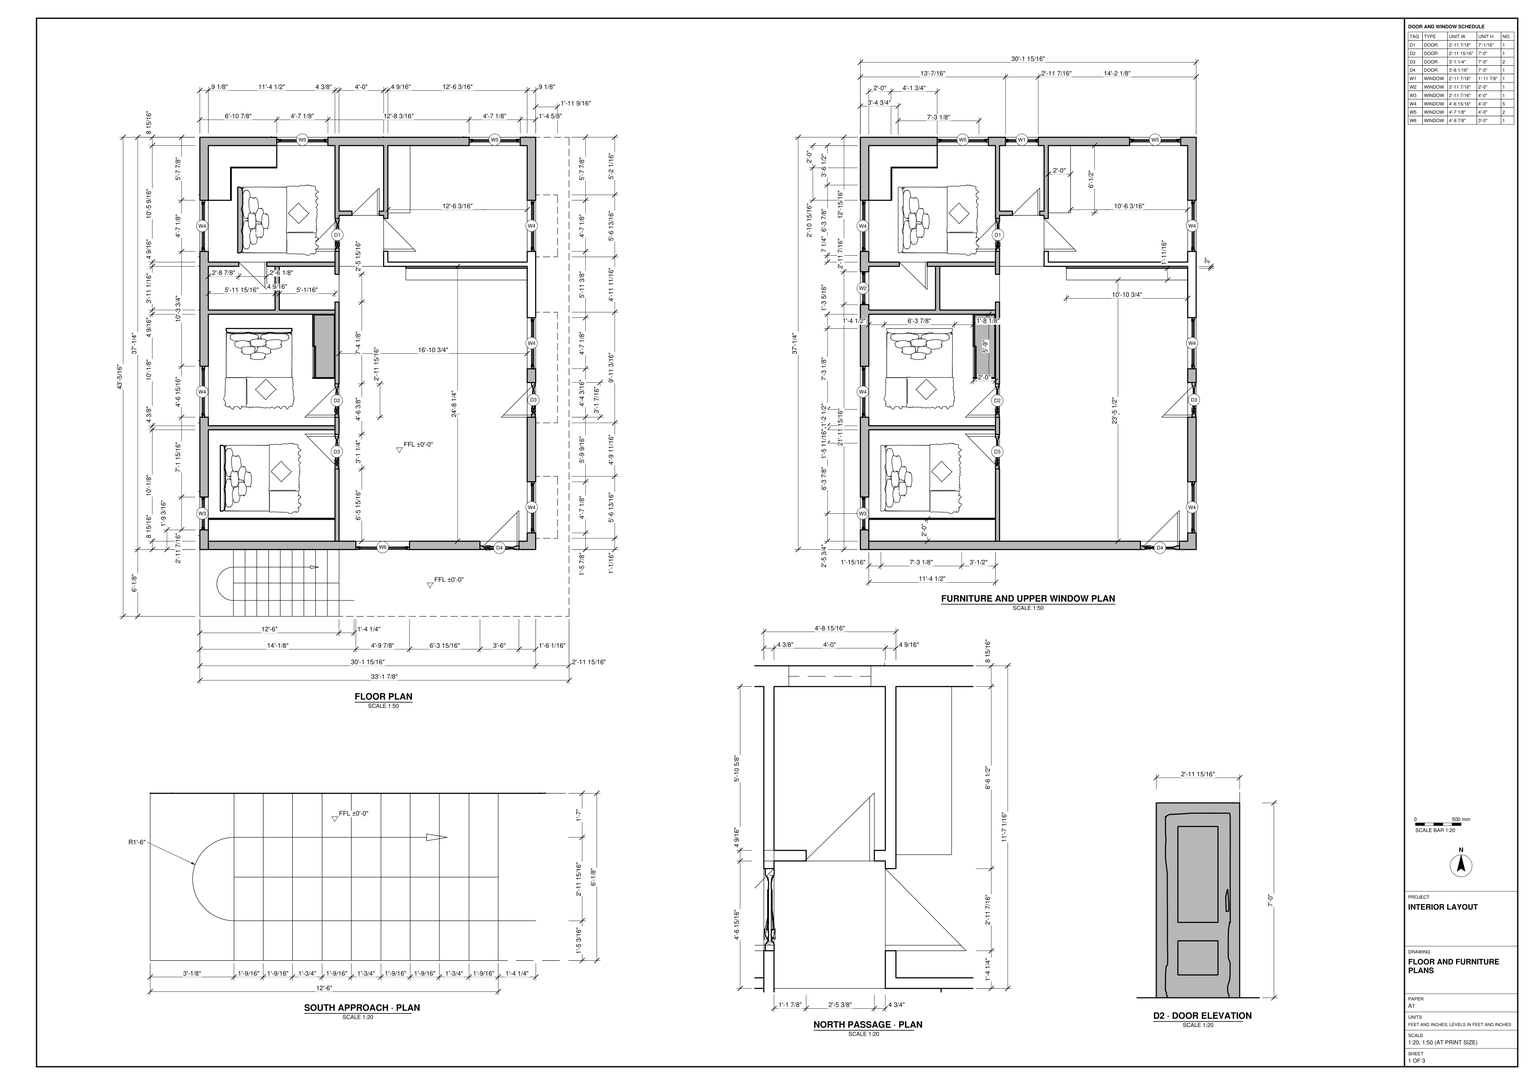
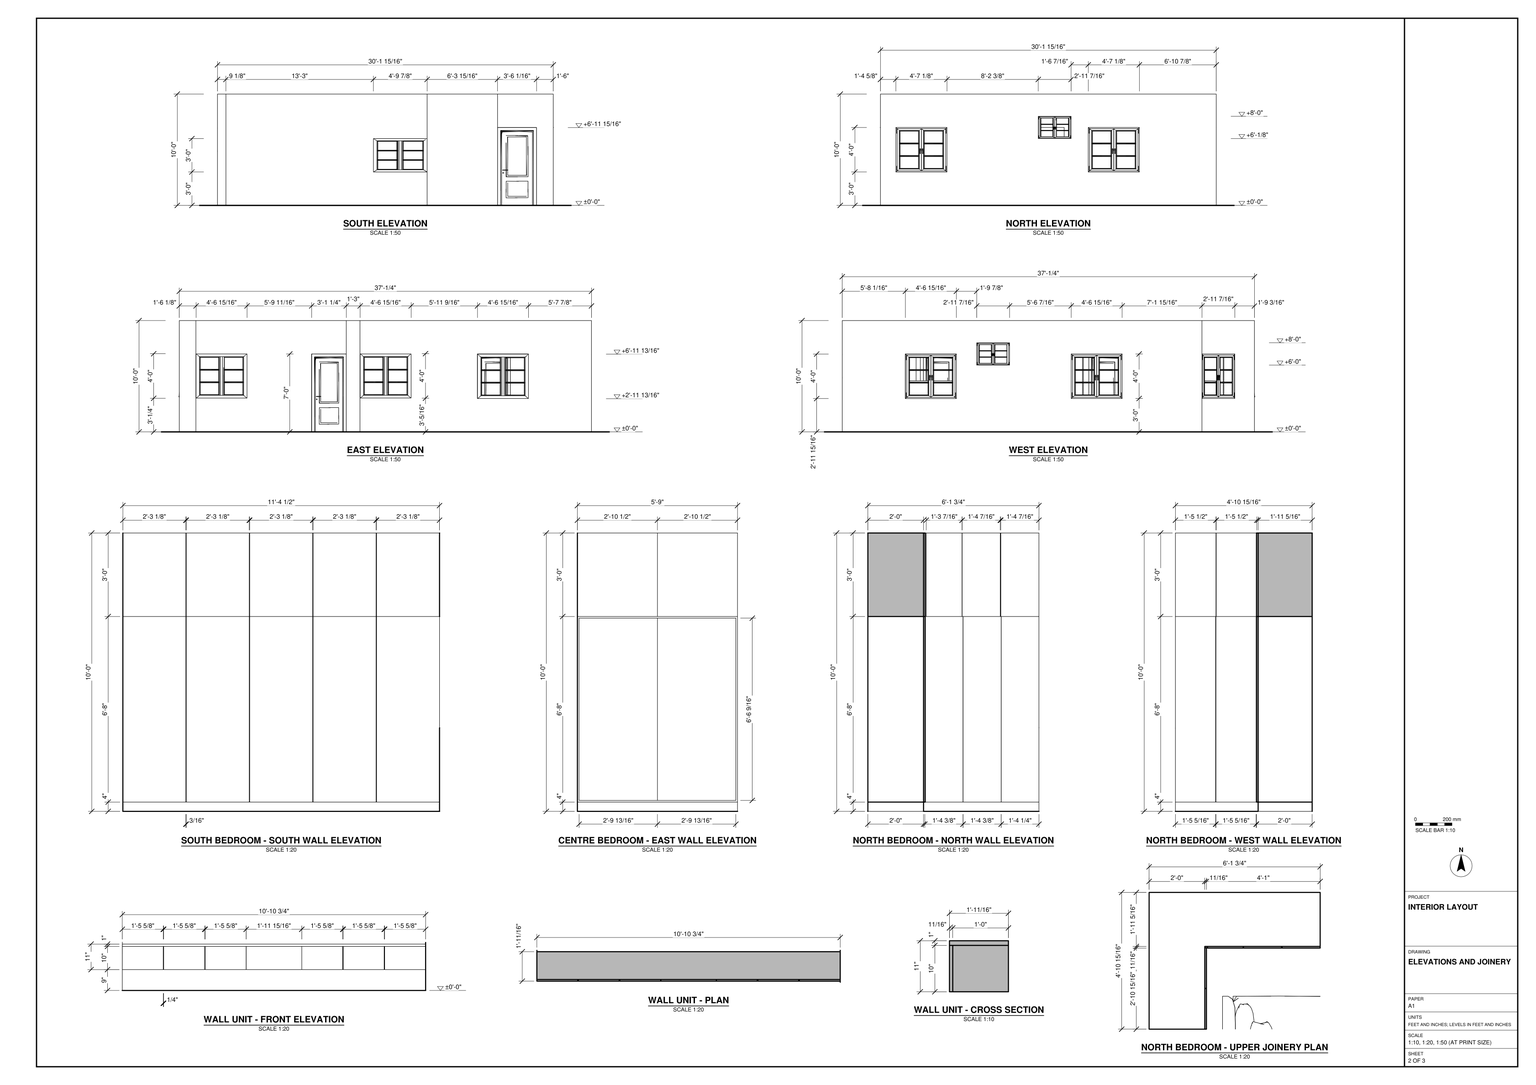
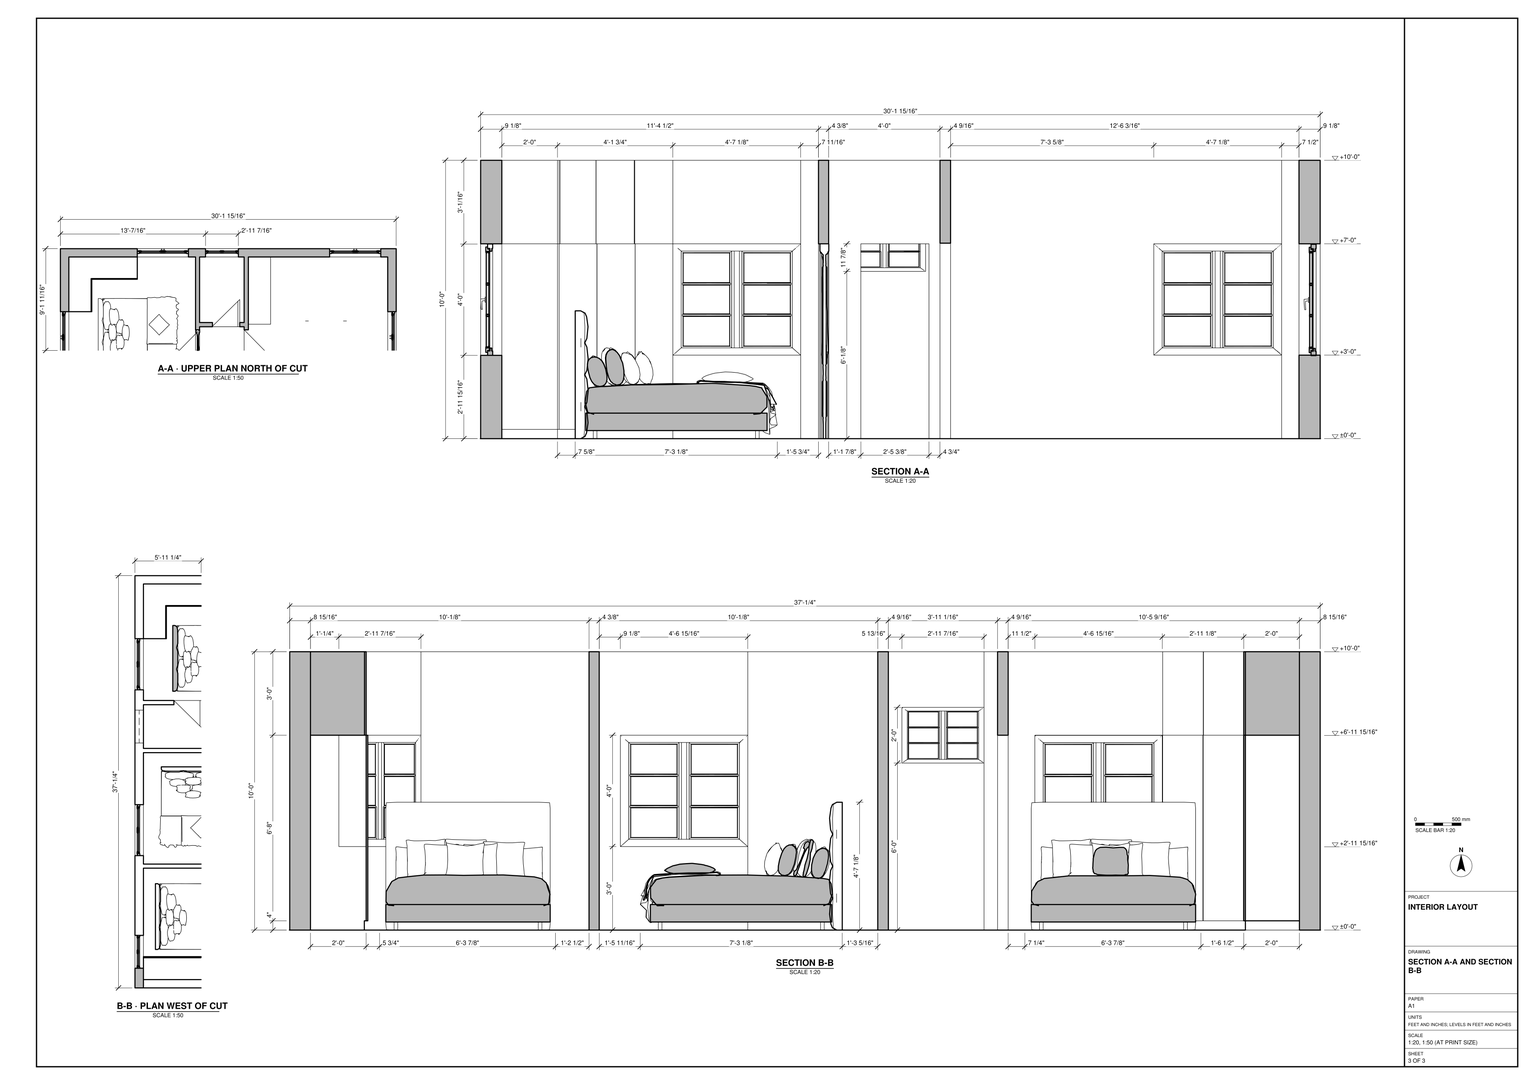
Build the single-storey interior in SketchUp from task_files/diagram_01.pdf. Work in feet and inches. The complete model extents are 120'-2 5/8" along X, 129'-1 1/8" along Y and 10'-1/16" along Z. These are not the room dimensions: use the dimensioned floor plan for the shell, which measures 30'-1 15/16" east to west by 37'-1/4" north to south. Set the finished floor level to ±0'-0".

Model the floor, perimeter walls and internal partitions using the individual wall thicknesses shown in plan. Arrange the three bedrooms along the west side, retaining the small space between the north and centre bedrooms, the narrow north passage and the large open room to the east. Include the divided south approach. Fit the doors and windows into wall openings; use the plans for door swings and the elevations and sections for sill heights, frames and window divisions. Note the smaller, higher windows on the north and west walls.

Place a bed in each bedroom with the footprint and orientation shown. Model the fitted storage along the south bedroom's south wall and the centre bedroom's east wall, and use the upper joinery plan for the corner storage in the north bedroom. Include the low wall unit in the large open room. Match the cabinet divisions to the joinery elevations. Decor and loose items may be any suitable library components.

Keep the shell elements and each furniture or joinery piece in separate groups or components, and use components for repeated parts. Save one SketchUp model as output_files/three_bedroom_interior_with_its_fitted_storage.skp.

# SketchUp Ruby script. Lengths in inches.
U = 1.inch
M = Sketchup.active_model
def pt(a) = Geom::Point3d.new(a.map { |v| v * U })
def face(e, loops, mat)
  f = e.add_face(loops[0].map { |a| pt(a) })
  loops[1..].each { |l| e.add_face(l.map { |a| pt(a) }).erase! }
  f.material = f.back_material = mat if mat
  f
end
# faces: each face lists its corners as indices into pts; further lists are holes
def faces(e, pts, list, mat = nil) = list.each { |f| face(e, (f[0].is_a?(Array) ? f : [f]).map { |l| l.map { |i| pts[i] } }, mat) }
# xy, xz, yz: faces in a plane at the given z, y or x. An outline is a flat list of corners, or four numbers for a rectangle; further outlines are holes
def ring(l) = l.size == 4 ? [[l[0], l[1]], [l[2], l[1]], [l[2], l[3]], [l[0], l[3]]] : l.each_slice(2).to_a
def flat(e, list, mat, &to3) = list.each { |f| face(e, (f[0].is_a?(Array) ? f : [f]).map { |l| ring(l).map { |u, v| to3.(u, v) } }, mat) }
def xy(e, z, list, mat = nil) = flat(e, list, mat) { |x, y| [x, y, z] }
def xz(e, y, list, mat = nil) = flat(e, list, mat) { |x, z| [x, y, z] }
def yz(e, x, list, mat = nil) = flat(e, list, mat) { |y, z| [x, y, z] }
def lines(e, pts, list) = list.each { |a, b| e.add_line(pt(pts[a]), pt(pts[b])) }
# prism: a flat outline (further loops are holes) pulled along v
def prism(e, loops, v, mat = nil)
  f = face(e, loops, mat); d = Geom::Vector3d.new(v.map { |x| x * U })
  f.pushpull(f.normal.samedirection?(d) ? d.length : -d.length)
end
def box(e, o, s, mat = nil) = prism(e, [[o, [o[0] + s[0], o[1], o[2]], [o[0] + s[0], o[1] + s[1], o[2]], [o[0], o[1] + s[1], o[2]]]], [0, 0, s[2]], mat)
def at(x, y, z, deg = 0) = Geom::Transformation.translation(pt([x, y, z])) * Geom::Transformation.rotation(ORIGIN, Z_AXIS, deg.degrees)
def axes(o, x, y, z) = Geom::Transformation.new([*x, 0, *y, 0, *z, 0, *pt(o).to_a, 1])
def part(name) = M.definitions.add(name)
# library, detail: a bought-in or finely detailed component or shape, given as its bounding box
def library(name, o, s) = part(name).tap { |d| box(d.entities, o, s) }
def detail(e, o, s) = box(e.add_group.entities, o, s)
def put(e, d, t, mat = nil) = e.add_instance(d, t).tap { |i| i.material = mat if mat }
def group(e, t, mat = nil) = e.add_group.tap { |g| g.transformation = t; g.material = mat if mat }.entities
root = M.entities
M.materials.add("[0007_MistyRose]").color = [255, 228, 225]
M.materials.add("[Basic Tile]").color = [203, 206, 207]
M.materials.add("[Color M00]").color = [255, 255, 255]
M.materials.add("[Concrete Tile]").color = [203, 190, 164]
M.materials.add("[Granite Tile]").color = [155, 148, 143]
M.materials.add("[Marble Carrara Gold Floor Tile]").color = [225, 223, 217]
M.materials.add("[Terrazzo Tile Accent]").color = [224, 221, 217]
c1 = part("29 cad.dwg")
xy(c1.entities,0,[[6.02,61.14,4.38,70.09,7.48,70.09],[174.3,112.79,174.3,115.72,183.25,114.26],[4.38,124.11,6.02,133.24,7.48,124.11],[6.02,133.24,4.38,142.18,7.48,142.18],[4.38,568.54,6.02,577.48,7.48,568.54],
  [823.51,569.27,826.98,569.82,830.45,569.27],[64.25,629.68,55.12,631.14,64.25,632.78],[407.92,629.68,407.92,632.78,417.05,631.14],[425.99,629.68,417.05,631.14,425.99,632.78],[444.0625,629.68,444.0625,632.78,453.01,631.14]])
# 826 loose lines left out
c2 = library("Bed 003",[-38.05,-87.1,0],[75.86,87.1,55.12])
c3 = library("Window 46-30",[-29.96,-2.6,0],[59.92,5.19,59.84])
c4 = library("Door 243 074",[-20.11,-2.41,0],[40.22,4.82,86.63])
c5 = part("Group\#6")
box(c5.entities,[0,0,0],[0.71,34.51,36])
c6 = part("Group\#13")
box(c6.entities,[0,0.16,0],[0.71,17.32,80])
c7 = part("Group\#14")
box(c7.entities,[0,1.07,0],[0.71,16.41,80])
c8 = part("Group\#18")
box(c8.entities,[0,0,0],[16.42,0.71,36])
c9 = part("Group\#17")
box(c9.entities,[-1.05,0,0],[17.47,0.71,36])
c10 = part("Group\#10")
box(c10.entities,[0,0,0],[17.64,0.71,10])
c11 = part("Group\#19")
box(c11.entities,[0.16,0,0],[27.14,0.71,80],"[Color M00]")
c12 = part("Group\#21")
box(c12.entities,[0.16,0,0],[27.14,0.71,36],"[Color M00]")
xy(root,0,[[398.98,439.99,417.05,439.99,417.05,582.53,407.92,582.53,407.92,448.93,398.98,448.93],[200.77,448.93,205.15,526.86],[55.12,496.57,64.25,496.57,64.25,569.03,200.77,569.03,200.77,573.41,64.25,573.41,64.25,637.47,55.12,637.47],[200.77,564.09,205.15,582.53],[200.77,618.49,205.15,706.64],
  [407.92,619.95,417.05,619.95,417.05,884.23,55.12,884.23,55.12,739.3125,64.25,739.3125,64.25,745.15,97.1,745.15,97.1,749.72,64.25,749.72,64.25,875.29,200.77,875.29,200.77,804.65,205.15,804.65,205.15,875.29,253.15,875.29,253.15,804.65,248.4,804.65,248.4,800.09,253.15,800.09,253.15,796.81,257.71,796.81,257.71,875.29,407.92,875.29,407.92,749.72,257.71,749.72,257.71,761.4,253.15,761.4,253.15,745.15,407.92,745.15],[176.77,624.49,200.77,693.5],[55.12,637.47,64.25,637.47,64.25,693.5,200.77,693.5,200.77,698.06,140.72,698.06,140.72,745.15,136.16,745.15,136.16,698.06,64.25,698.06,64.25,739.3125,55.12,739.3125],[200.77,736.58,205.15,761.4],[277.15,743.15,407.92,745.15],
  [127.21,745.15,200.77,749.72],[200.77,796.81,205.15,800.09],[200.77,800.09,205.15,804.65],[205.15,800.09,219.02,804.65]])
xy(root,0,[[[0,0,1442.625,1549.125],[398.98,439.99,398.98,448.93,64.25,448.93,64.25,472.93,200.77,472.93,200.77,526.86,205.15,526.86,205.15,564.09,200.77,564.09,200.77,569.03,64.25,569.03,64.25,496.57,55.12,496.57,55.12,884.23,417.05,884.23,417.05,619.95,407.92,619.95,407.92,582.53,417.05,582.53,417.05,439.99]]],"[0007_MistyRose]")
xy(root,0,[[64.25,749.72,200.77,749.72,200.77,875.29,137.98,875.29,137.98,852,88.25,852,88.25,816.34,64.25,816.34],[200.77,761.4,205.15,796.81]],"[Basic Tile]")
xy(root,0,[[64.25,448.93,200.77,472.93]],"[Color M00]")
xy(root,0,[[219.02,800.09,248.4,800.09,248.4,804.65,253.15,804.65,253.15,875.29,205.15,875.29,205.15,804.65,219.02,804.65]],"[Concrete Tile]")
xy(root,0,[[257.71,749.72,407.92,749.72,407.92,875.29,281.71,875.29,281.71,802.81,257.71,802.81,257.71,796.81,253.15,796.81,253.15,761.4,257.71,761.4],[257.71,802.81,281.71,875.29]],"[Granite Tile]")
xy(root,0,[[205.15,448.93,407.92,448.93,407.92,743.15,277.15,743.15,277.15,745.15,205.15,745.15],[205.15,745.15,253.15,800.09]],"[Marble Carrara Gold Floor Tile]")
xy(root,0,[[64.25,573.41,200.77,573.41,200.77,582.53,205.15,582.53,205.15,618.49,200.77,618.49,200.77,624.49,176.77,624.49,176.77,693.5,64.25,693.5],[64.25,698.06,136.16,698.06,136.16,745.15,127.21,745.15,127.21,749.72,97.1,749.72,97.1,745.15,64.25,745.15],[140.72,698.06,200.77,698.06,200.77,706.64,205.15,706.64,205.15,736.58,200.77,736.58,200.77,745.15,140.72,745.15]],"[Terrazzo Tile Accent]")
xy(root,4,[[64.25,816.34,64.25,875.29,137.98,875.29,137.98,852,88.25,852,88.25,816.34]])
xy(root,35.92,[[55.12,761.22,64.25,816.34]])
xy(root,36,[[55.12,582.53,64.25,637.47],[407.92,761.22,417.05,816.34],[137.98,875.29,193.1,884.23],[345.32,875.29,400.44,884.23]])
xy(root,36.44,[[407.92,457.875,417.05,512.99]])
xy(root,36.52,[[407.92,634.73,417.05,689.85]])
xy(root,72,[[55.12,703.91,64.25,739.3125]])
xy(root,72.11,[[211.54,875.29,246.94,884.23]])
xy(root,84,[[357,439.99,398.98,448.93],[407.92,457.875,417.05,512.99],[200.77,526.86,205.15,564.09],[55.12,582.53,64.25,637.47],[200.77,582.53,205.15,618.49],
  [407.92,582.53,417.05,619.95],[407.92,634.73,417.05,689.85],[200.77,706.64,205.15,736.58],[97.1,745.15,127.21,749.72],[127.21,745.15,136.16,749.72],
  [55.12,761.22,64.25,816.34],[407.92,761.22,417.05,816.34],[200.77,761.4,205.15,796.81],[219.02,800.09,248.4,804.65],[64.25,816.34,88.25,816.34,88.25,852,137.98,852,137.98,875.29,64.25,875.29],
  [137.98,875.29,193.1,884.23],[345.32,875.29,400.44,884.23]])
xy(root,84.27,[[253.15,761.4,257.71,796.81]])
xy(root,96,[[55.12,703.91,64.25,739.3125],[211.54,875.29,246.94,884.23]])
xy(root,120,[[[357,439.99,417.05,439.99,417.05,884.23,55.12,884.23,55.12,496.57,64.25,496.57,64.25,745.15,136.16,745.15,136.16,749.72,64.25,749.72,64.25,875.29,253.15,875.29,253.15,804.65,205.15,804.65,205.15,875.29,200.77,875.29,200.77,761.4,205.15,761.4,205.15,800.09,253.15,800.09,253.15,745.15,407.92,745.15,407.92,448.93,357,448.93],[257.71,749.72,407.92,875.29]],[200.77,448.93,205.15,582.53],[64.25,569.03,200.77,573.41],[200.77,582.53,205.15,761.4],[64.25,693.5,200.77,693.5,200.77,698.06,140.72,698.06,140.72,745.15,136.16,745.15,136.16,698.06,64.25,698.06],
  [277.28,743.15,407.92,745.15],[136.16,745.15,200.77,749.72]])
xz(root,439.99,[[398.98,0,417.05,0,417.05,120,357,120,357,84,398.98,84]])
xz(root,448.93,[[200.77,0,205.15,120],[398.98,0,398.98,84,357,84,357,120,407.92,120,407.92,0]])
xz(root,457.875,[[407.92,36.44,417.05,84]])
xz(root,496.57,[[55.12,0,64.25,120]])
xz(root,512.99,[[407.92,36.44,417.05,84]])
xz(root,526.86,[[200.77,0,205.15,84]])
xz(root,564.09,[[200.77,0,205.15,84]])
xz(root,569.03,[[64.25,0,200.77,120]])
xz(root,573.41,[[64.25,0,200.77,120]])
xz(root,582.53,[[200.77,0,205.15,84],[407.92,0,417.05,84],[55.12,36,64.25,84]])
xz(root,618.49,[[200.77,0,205.15,84]])
xz(root,619.95,[[407.92,0,417.05,84]])
xz(root,634.73,[[407.92,36.52,417.05,84]])
xz(root,637.47,[[55.12,36,64.25,84]])
xz(root,689.85,[[407.92,36.52,417.05,84]])
xz(root,693.5,[[64.25,0,200.77,120]])
xz(root,698.06,[[64.25,0,136.16,120],[140.72,0,200.77,120]])
xz(root,703.91,[[55.12,72,64.25,96]])
xz(root,706.64,[[200.77,0,205.15,84]])
xz(root,736.58,[[200.77,0,205.15,84]])
xz(root,737.15,[[407.92,87.4,407.92,88.4,277.25,88.55,277.25,87.55]])
xz(root,739.3125,[[55.12,72,64.25,96]])
xz(root,743.15,[[277.15,0,407.92,0,407.92,87.4,277.25,87.55],[407.92,88.4,407.92,120,277.28,120,277.25,88.55]])
xz(root,745.15,[[64.25,0,97.1,0,97.1,84,136.16,84,136.16,120,64.25,120],[127.21,0,136.16,84],[136.16,0,140.72,120],[140.72,0,200.77,120],[253.15,0,277.15,0,277.28,120,253.15,120],
  [277.15,0,277.28,120,407.92,120,407.92,0]])
xz(root,749.72,[[64.25,0,64.25,120,136.16,120,136.16,84,97.1,84,97.1,0],[127.21,0,127.21,84,136.16,84,136.16,120,200.77,120,200.77,0],[257.71,0,407.92,120]])
xz(root,761.22,[[55.12,35.92,64.25,84],[407.92,36,417.05,84]])
xz(root,761.4,[[200.77,0,205.15,84],[253.15,0,257.71,84.27]])
xz(root,796.81,[[200.77,0,205.15,84],[253.15,0,257.71,84.27]])
xz(root,800.09,[[205.15,0,219.02,0,219.02,84,248.4,84,248.4,0,253.15,0,253.15,120,205.15,120]])
xz(root,804.65,[[205.15,0,205.15,120,248.4,120,248.4,84,219.02,84,219.02,0],[248.4,0,253.15,120]])
xz(root,816.34,[[64.25,0,88.25,4],[64.25,4,88.25,84],[55.12,35.92,64.25,84],[407.92,36,417.05,84]])
xz(root,852,[[88.25,0,137.98,4],[88.25,4,104.82,84],[104.82,4,121.4,84],[121.4,4,137.98,84]])
xz(root,875.29,[[64.25,0,137.98,4],[137.98,0,193.1,36],[193.1,0,200.77,120],[[205.15,0,253.15,120],[211.54,72.11,246.94,96]],[257.71,0,400.44,0,400.44,36,345.32,36,345.32,84,400.44,84,400.44,120,257.71,120],
  [400.44,0,407.92,120],[64.25,4,137.98,84],[64.25,84,193.1,120]])
xz(root,884.23,[[[55.12,0,417.05,120],[137.98,36,193.1,84],[345.32,36,400.44,84],[211.54,72.11,246.94,96]]])
yz(root,55.12,[[[496.57,0,884.23,120],[761.22,35.92,816.34,84],[582.53,36,637.47,84],[703.91,72,739.3125,96]]])
yz(root,64.25,[[496.57,0,569.03,120],[573.41,0,637.47,0,637.47,36,582.53,36,582.53,84,637.47,84,637.47,120,573.41,120],[637.47,0,693.5,120],[698.06,0,739.3125,0,739.3125,72,703.91,72,703.91,96,739.3125,96,739.3125,120,698.06,120],[739.3125,0,745.15,120],
  [749.72,0,816.34,0,816.34,35.92,761.22,35.92,761.22,84,875.29,84,875.29,120,749.72,120],[816.34,0,875.29,4],[816.34,4,875.29,84]])
yz(root,88.25,[[816.34,0,852,4],[816.34,4,833.8125,84],[833.8125,4,852,84]])
yz(root,97.1,[[745.15,0,749.72,84]])
yz(root,127.21,[[745.15,0,749.72,84]])
yz(root,136.16,[[698.06,0,745.15,120],[745.15,84,749.72,120]])
yz(root,137.98,[[852,0,875.29,4],[852,4,875.29,84],[875.29,36,884.23,84]])
yz(root,140.72,[[698.06,0,745.15,120]])
yz(root,193.1,[[875.29,36,884.23,84]])
yz(root,200.77,[[448.93,0,448.93,120,569.03,120,569.03,0,564.09,0,564.09,84,526.86,84,526.86,0],[569.03,0,573.41,120],[573.41,0,582.53,120],[618.49,0,618.49,84,582.53,84,582.53,120,693.5,120,693.5,0],[693.5,0,698.06,120],
  [698.06,0,698.06,120,745.15,120,745.15,0,736.58,0,736.58,84,706.64,84,706.64,0],[745.15,0,749.72,120],[749.72,0,761.4,120],[796.81,0,796.81,84,761.4,84,761.4,120,800.09,120,800.09,0],[800.09,0,804.65,120],
  [804.65,0,875.29,120]])
yz(root,205.15,[[448.93,0,526.86,0,526.86,84,564.09,84,564.09,0,582.53,0,582.53,120,448.93,120],[618.49,0,706.64,0,706.64,84,736.58,84,736.58,0,761.4,0,761.4,120,582.53,120,582.53,84,618.49,84],[796.81,0,800.09,0,800.09,120,761.4,120,761.4,84,796.81,84],[804.65,0,875.29,120]])
yz(root,211.54,[[875.29,72.11,884.23,96]])
yz(root,219.02,[[800.09,0,804.65,84]])
yz(root,246.94,[[875.29,72.11,884.23,96]])
yz(root,248.4,[[800.09,0,804.65,84]])
yz(root,253.15,[[745.15,0,745.15,120,800.09,120,800.09,0,796.81,0,796.81,84.27,761.4,84.27,761.4,0],[804.65,0,875.29,120]])
yz(root,257.71,[[749.72,0,761.4,0,761.4,84.27,796.81,84.27,796.81,0,875.29,0,875.29,120,749.72,120]])
yz(root,277.25,[[737.15,87.55,743.15,88.55]])
yz(root,345.32,[[875.29,36,884.23,84]])
yz(root,357,[[439.99,84,448.93,120]])
yz(root,398.98,[[439.99,0,448.93,84]])
yz(root,400.44,[[875.29,36,884.23,84]])
yz(root,407.92,[[[448.93,0,448.93,120,743.15,120,743.15,0,619.95,0,619.95,84,582.53,84,582.53,0],[457.875,36.44,512.99,84],[634.73,36.52,689.85,84]],[743.15,0,743.15,87.4,745.15,120,745.15,0],[[749.72,0,875.29,120],[761.22,36,816.34,84]],[737.15,87.4,743.15,88.4],[743.15,87.4,743.15,88.4,745.15,120],
  [743.15,88.4,743.15,120,745.15,120]])
yz(root,417.05,[[439.99,0,457.875,120],[457.875,0,582.53,0,582.53,84,619.95,84,619.95,120,457.875,120,457.875,84,512.99,84,512.99,36.44,457.875,36.44],[619.95,0,634.73,120],[[634.73,0,884.23,0,884.23,120,634.73,120,634.73,84,689.85,84,689.85,36.52,634.73,36.52],[761.22,36,816.34,84]]])
# 1 loose lines left out
p = [[277.25,743.15,87.55],[277.28,745.15,120],[277.15,745.15,0],[277.15,743.15,0],[407.92,743.15,87.4],[407.92,737.15,87.4],
  [277.25,737.15,87.55],[277.25,743.15,88.55],[407.92,743.15,88.4],[277.25,737.15,88.55],[407.92,737.15,88.4],[277.28,743.15,120]]
faces(root,p,[[0,1,2,3],[0,4,5,6],[0,7,1],[8,7,9,10],[11,1,7]])
put(root,c1,at(0,306.75,0))
put(root,c2,at(118.83,678.1875,0))
put(root,c3,axes([57.72,610,36],[0,-0.91688,0],[1,0,0],[0,0,0.80216]))
put(root,c3,axes([57.72,478.86,36],[0,-0.59095,0],[1,0,0],[0,0,0.80216]))
put(root,c3,axes([57.72,788.68,35.92],[0,-0.91688,0],[1,0,0],[0,0,0.80216]))
put(root,c3,axes([57.72,721.61,72],[0,-0.59095,0],[1,0,0],[0,0,0.40108]))
put(root,c3,axes([165.54,881.63,36],[-0.91993,0,0],[0,-1,0],[0,0,0.80216]))
put(root,c3,axes([229.24,881.63,72.1],[-0.59095,0,0],[0,-1,0],[0,0,0.39932]))
put(root,c3,axes([372.88,881.63,36],[-0.91993,0,0],[0,-1,0],[0,0,0.80216]))
put(root,c3,axes([412.71,788.91,35.79],[0,-0.91688,0],[1,0,0],[0,0,0.80216]))
put(root,c3,axes([412.71,662.42,36.31],[0,-0.91688,0],[1,0,0],[0,0,0.80216]))
put(root,c3,axes([412.71,485.5625,36.23],[0,-0.91688,0],[1,0,0],[0,0,0.80216]))
put(root,c3,axes([252.15,442.58,36],[-0.96562,0,0],[0,-1,0],[0,0,0.60162]))
put(root,c4,axes([202.74,600.51,0],[0,0.8938,0],[-1,0,0],[0,0,0.9696]))
put(root,c4,axes([202.74,545.48,0],[0,0.92532,0],[-1,0,0],[0,0,0.9696]))
put(root,c4,axes([203.375,779.1,-0.0625],[0,0.88018,0],[-1,0,0],[0,0,0.97034]))
put(root,c2,at(77.18,516.75,0,90))
put(root,c2,at(95.89,795,0,90))
put(root,c4,axes([414.64,601.34,0],[0,0.92532,0],[-1,0,0],[0,0,0.9696]))
put(root,c4,axes([378.02,441.83,-0.07],[1.04502,0,0],[0,1,0],[0,0,0.9696]))
g1 = group(root,at(64.25,439.99,0))
xy(g1,0,[[-9.125,0,0,56.58],[0,0,216.83,8.94],[216.83,0,292.76,8.94]])
xy(g1,36,[[158.97,0,216.83,8.94],[-9.125,21.17,0,56.58]])
xy(g1,72,[[158.97,0,216.83,8.94]])
xy(g1,84,[[-9.125,21.17,0,56.58]])
xy(g1,120,[[-9.125,0,0,56.58],[0,0,292.76,8.94]])
xz(g1,0,[[-9.125,0,0,120],[0,0,216.83,0,216.83,36,158.97,36,158.97,72,216.83,72,216.83,120,0,120],[216.83,0,292.76,120]])
xz(g1,8.94,[[[0,0,292.76,120],[158.97,36,216.83,72]]])
xz(g1,21.17,[[-9.125,36,0,84]])
xz(g1,56.58,[[-9.125,0,0,36],[-9.125,84,0,120]])
yz(g1,-9.125,[[0,0,0,120,56.58,120,56.58,84,21.17,84,21.17,36,56.58,36,56.58,0]])
yz(g1,0,[[0,0,8.94,120],[8.94,0,56.58,0,56.58,36,21.17,36,21.17,84,56.58,84,56.58,120,8.94,120]])
yz(g1,158.97,[[0,36,8.94,72]])
yz(g1,216.83,[[0,36,8.94,72]])
yz(g1,292.76,[[0,0,8.94,120]])
g2 = group(root,at(176.77,624.49,0))
g3 = group(g2,at(0,34.51,4.71))
box(g3,[0,0,0],[1.5,33.8,78.58])
g4 = group(g2,at(1.5,0.71,4.71))
box(g4,[0,0,0],[1.5,33.8,79.04])
g5 = group(g2,at(0,0,0))
xy(g5,0,[[0,0,24,69.01]])
xy(g5,4.71,[[0,0.71,23.29,0.71,23.29,68.31,3,68.31,3,34.51,1.5,34.51,1.5,68.31,0,68.31],[1.5,34.51,3,68.31]])
xy(g5,83.29,[[0,0.71,23.29,68.31]])
xy(g5,84,[[0,0,24,69.01]])
xz(g5,0,[[0,0,24,84]])
xz(g5,0.71,[[0,4.71,23.29,83.29]])
xz(g5,68.31,[[0,4.71,23.29,83.29]])
xz(g5,69.01,[[0,0,24,84]])
yz(g5,0,[[0,0,69.01,4],[[0,4,69.01,84],[0.71,4.71,68.31,83.29]]])
yz(g5,23.29,[[0.71,4.71,68.31,83.29]])
yz(g5,24,[[0,0,69.01,84]])
put(root,c5,at(176.77,658.99,84))
put(root,c5,at(176.77,624.49,84))
g6 = group(root,at(177.48,624.49,84))
prism(g6,[[[0,0,0],[0,34.51,0],[0,69.01,0],[23.29,69.01,0],[23.29,0,0]]],[0,0,36])
put(root,c6,at(88.25,816.18,4))
put(root,c6,at(88.25,833.65,4))
g7 = group(root,at(120.66,852,4,-90))
box(g7,[0,1.07,0],[0.71,16.25,80])
put(root,c7,at(104.22,852,4,-90))
put(root,c7,at(87.76,852,4,-90))
put(root,c8,at(121.5625,851.29,84))
g8 = group(root,at(64.25,816.34,84))
prism(g8,[[[24,35.66,0],[24,17.48,0],[24,0,0],[0,0,0],[0,58.95,0],[73.74,58.95,0],[73.74,35.66,0],[57.16,35.66,0],[40.58,35.66,0]]],[0,0,36])
put(root,c8,at(104.9,851.29,84))
g9 = group(root,at(89.4,851.29,84))
box(g9,[0,0,0],[15.42,0.71,36])
put(root,c9,at(88.95,834.99,84,90))
put(root,c9,at(88.95,817.39,84,90))
g10 = group(root,at(277.15,731.15,9))
prism(g10,[[[0,12,0],[130.77,12,0],[130.77,0,0],[112.98,0,0],[95.18,0,0],[77.39,0,0],[53.39,0,0],[0,0,0]]],[0,0,10])
put(g10,c10,at(113.14,-0.71,0))
put(g10,c10,at(95.26,-0.71,0))
put(g10,c10,at(77.39,-0.71,0))
put(g10,c10,at(0,-0.71,0))
put(g10,c10,at(35.75,-0.71,0))
put(g10,c10,at(17.875,-0.71,0))
g11 = group(g10,at(59.75,-0.71,0))
box(g11,[-6.3125,0,0],[23.95,0.71,10])
g12 = group(g10,at(0,0,10))
prism(g12,[[[0,12,0],[130.77,12,0],[130.77,-0.71,0],[0,-0.71,0],[0,0,0]]],[0,0,1])
# 6 loose lines left out
put(root,c11,at(91.55,473.64,4,-180))
g13 = group(root,at(200.77,472.93,0,-180))
xy(g13,0,[[0,0.79,136.52,24]],"[Color M00]")
xy(g13,4,[[0,0,136.52,0.79]],"[Color M00]")
xy(g13,84,[[0,0,136.52,24]],"[Color M00]")
xz(g13,0,[[0,4,109.22,84],[109.22,4,136.52,84]],"[Color M00]")
xz(g13,0.79,[[0,0,136.52,4]],"[Color M00]")
xz(g13,24,[[0,0,136.52,84]],"[Color M00]")
yz(g13,0,[[0.79,0,0.79,4,0,4,0,84,24,84,24,0]],"[Color M00]")
yz(g13,136.52,[[0.79,0,24,0,24,84,0,84,0,4,0.79,4]],"[Color M00]")
put(root,c11,at(118.89,473.64,4,-180))
put(root,c11,at(146.24,473.64,4,-180))
put(root,c11,at(173.58,473.64,4,-180))
put(root,c11,at(200.93,473.64,4,-180))
put(root,c12,at(64.09,472.22,84))
g14 = group(root,at(64.25,448.93,84))
xy(g14,0,[[0,0,136.52,23.29]],"[Color M00]")
xy(g14,36,[[0,0,136.52,23.29]],"[Color M00]")
xz(g14,0,[[0,0,136.52,36]],"[Color M00]")
xz(g14,23.29,[[0,0,109.22,36],[109.22,0,136.52,36]],"[Color M00]")
yz(g14,0,[[0,0,23.29,36]],"[Color M00]")
yz(g14,136.52,[[0,0,23.29,36]],"[Color M00]")
put(root,c12,at(118.78,472.22,84))
put(root,c12,at(146.12,472.22,84))
put(root,c12,at(173.46,472.22,84))
put(root,c12,at(91.43,472.22,84))
